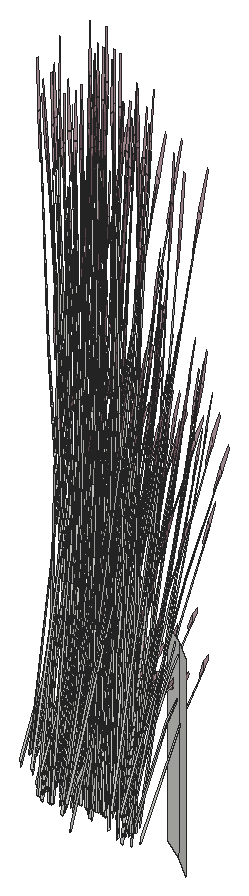
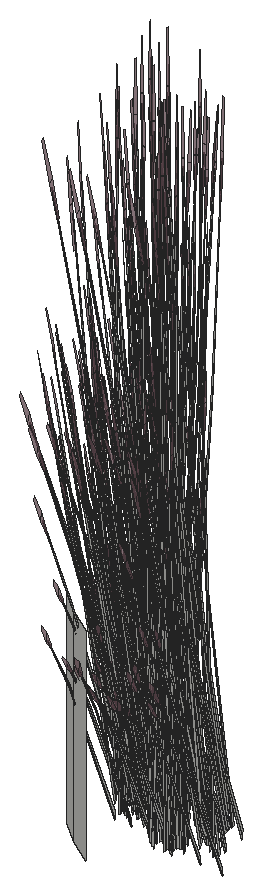
# SketchUp Ruby script. Lengths in inches.
U = 1.inch
M = Sketchup.active_model
def pt(a) = Geom::Point3d.new(a.map { |v| v * U })
def face(e, loops, mat)
  f = e.add_face(loops[0].map { |a| pt(a) })
  loops[1..].each { |l| e.add_face(l.map { |a| pt(a) }).erase! }
  f.material = f.back_material = mat if mat
  f
end
# faces: each face lists its corners as indices into pts; further lists are holes
def faces(e, pts, list, mat = nil) = list.each { |f| face(e, (f[0].is_a?(Array) ? f : [f]).map { |l| l.map { |i| pts[i] } }, mat) }
# xy, xz, yz: faces in a plane at the given z, y or x. An outline is a flat list of corners, or four numbers for a rectangle; further outlines are holes
def ring(l) = l.size == 4 ? [[l[0], l[1]], [l[2], l[1]], [l[2], l[3]], [l[0], l[3]]] : l.each_slice(2).to_a
def flat(e, list, mat, &to3) = list.each { |f| face(e, (f[0].is_a?(Array) ? f : [f]).map { |l| ring(l).map { |u, v| to3.(u, v) } }, mat) }
def xy(e, z, list, mat = nil) = flat(e, list, mat) { |x, y| [x, y, z] }
def xz(e, y, list, mat = nil) = flat(e, list, mat) { |x, z| [x, y, z] }
def yz(e, x, list, mat = nil) = flat(e, list, mat) { |y, z| [x, y, z] }
def lines(e, pts, list) = list.each { |a, b| e.add_line(pt(pts[a]), pt(pts[b])) }
# prism: a flat outline (further loops are holes) pulled along v
def prism(e, loops, v, mat = nil)
  f = face(e, loops, mat); d = Geom::Vector3d.new(v.map { |x| x * U })
  f.pushpull(f.normal.samedirection?(d) ? d.length : -d.length)
end
def box(e, o, s, mat = nil) = prism(e, [[o, [o[0] + s[0], o[1], o[2]], [o[0] + s[0], o[1] + s[1], o[2]], [o[0], o[1] + s[1], o[2]]]], [0, 0, s[2]], mat)
def at(x, y, z, deg = 0) = Geom::Transformation.translation(pt([x, y, z])) * Geom::Transformation.rotation(ORIGIN, Z_AXIS, deg.degrees)
def axes(o, x, y, z) = Geom::Transformation.new([*x, 0, *y, 0, *z, 0, *pt(o).to_a, 1])
def part(name) = M.definitions.add(name)
# library, detail: a bought-in or finely detailed component or shape, given as its bounding box
def library(name, o, s) = part(name).tap { |d| box(d.entities, o, s) }
def detail(e, o, s) = box(e.add_group.entities, o, s)
def put(e, d, t, mat = nil) = e.add_instance(d, t).tap { |i| i.material = mat if mat }
def group(e, t, mat = nil) = e.add_group.tap { |g| g.transformation = t; g.material = mat if mat }.entities
root = M.entities
M.materials.add("LightPink_Translucent").color = [144, 107, 117]
M.materials["LightPink_Translucent"].alpha = 0.75
c1 = part("blade")
p = [[2.15,0.21,22],[0,0.17,0],[0.09,0.45,0],[2.18,0.31,22],[2.29,0.31,22],[0.38,0.45,0],
  [2.48,0.24,33],[2.49,0.24,33],[2.48,0.22,33]]
faces(c1.entities,p,[[0,1,2,3],[4,5,2,3],[6,3,4,7],[8,0,3,6]])
c2 = part("seeds")
p = [[0.3,-0.1,1.38],[-0.01,-0.03,1.59],[-0.01,-0.03,0.03],[0.14,-0.07,-0.07],[0.29,-0.03,3],[0.15,0.01,3.11]]
faces(c2.entities,p,[[0,1,2,3],[1,0,4,5]],"LightPink_Translucent")
c3 = part("blade with seeds")
put(c3.entities,c1,at(0,0,0))
put(c3.entities,c2,axes([2.4,0.25,30.99],[1.5799,-0.05474,1.17369],[-0.12525,1.92788,0.29478],[-0.07173,-0.02425,1.56792]))
p = [[367.36,357.2,618],[369.42,355.39,618],[369.42,355.39,636],[367.36,357.2,636],[365.07,358.73,618],[365.07,358.73,636]]
faces(root,p,[[0,1,2,3],[4,0,3,5]])
put(root,c3,axes([354.65,355.82,623.05],[-0.20082,-0.29199,0.35414],[0.2293,-0.2764,-0.4572],[0.1165,0.04206,0.87481]))
put(root,c3,axes([355.86,357.4,623.65],[0.2439,-0.26754,-0.06488],[0.22348,0.29302,-0.29416],[0.01573,0.08303,0.97024]))
put(root,c3,axes([358.69,356.23,620.06],[-0.23773,0.35053,-0.62353],[-0.29532,-0.31785,-0.16365],[-0.09526,0.08744,1.37633]))
put(root,c3,axes([354.83,356.09,622.73],[-0.01777,0.35463,0.0643],[-0.26836,-0.00972,0.50621],[0.1028,0.03711,0.77189]))
put(root,c3,axes([358.5,356.01,622.73],[-0.08753,-0.42921,0.48003],[0.34336,-0.07449,0.3958],[-0.1012,0.10094,0.9933]))
put(root,c3,axes([356.14,355.7,620.2],[0.35581,0.20937,0],[-0.17124,0.43505,0],[0,0,1.74954]))
put(root,c3,axes([354.76,356.64,619.49],[0.02571,-0.06733,1.76342],[0.32373,-0.19829,-0.26939],[0.09815,0.10263,0.30037]))
put(root,c3,axes([354.86,355.98,622.73],[-0.26024,0.30729,0.48003],[-0.22444,-0.32634,0.3958],[0.1221,0.05668,0.9933]))
put(root,c3,axes([358.4375,355.93,622.73],[-0.2423,-0.19613,0.0643],[0.14107,-0.2793,0.50621],[-0.07768,0.0903,0.77189]))
put(root,c3,axes([358.85,356.03,620.46],[-0.34464,-0.37536,-0.25192],[0.29,-0.42149,0.5513],[-0.0928,0.04391,1.68216]))
put(root,c3,axes([357.19,354.89,620.03],[-0.24637,0.29097,-0.30978],[-0.24637,-0.29097,0.30978],[0,0.09372,1.38974]))
put(root,c3,axes([356.49,354.84,620.09],[0.12941,0.42699,-0.69212],[-0.37279,0.15378,-0.18165],[0.0143,0.14459,1.52773]))
put(root,c3,axes([358.68,355.95,620.21],[-0.38326,0.02879,-0.44739],[-0.03466,-0.47788,0.21531],[-0.06861,0.04843,1.43643]))
put(root,c3,axes([358.72,356.14,622.68],[0.09067,0.42583,-0.51099],[-0.34336,0.07449,-0.3958],[-0.0984,0.11438,0.97773]))
put(root,c3,axes([357.95,356.75,620.48],[0.33032,0.23318,0.49651],[-0.19744,0.41812,0],[-0.07523,-0.05311,1.57504]))
put(root,c3,axes([356.33,354.36,620.67],[0.39748,0.22252,-0.29095],[-0.19139,0.46966,-0.50002],[0.01249,0.11531,1.59708]))
put(root,c3,axes([354.22,355.23,621.875],[-0.1311,-0.08035,1.71376],[0.27131,-0.33708,0.13857],[0.16909,0.15206,0.73262]))
put(root,c3,axes([359.08,357.1875,620.02],[-0.33032,0.23318,-0.49651],[-0.19744,-0.41812,0],[-0.07523,0.05311,1.57504]))
put(root,c3,axes([359.1,357.0625,620.19],[-0.21791,-0.46895,-0.05142],[0.36918,-0.26061,0.51607],[-0.09097,0.04465,1.6363]))
put(root,c3,axes([357.36,354.9,620.02],[0,0.46636,-0.49651],[-0.39487,0,0],[0,0.10622,1.57504]))
put(root,c3,axes([356.31,356.32,622.73],[-0.35104,0.10702,0.48003],[-0.06092,-0.41983,0.3958],[0.08256,0.12373,0.9933]))
put(root,c3,axes([354.9375,355.98,622.53],[0.20082,0.29199,-0.35414],[-0.2293,0.2764,0.4572],[0.1165,0.04206,0.87481]))
put(root,c3,axes([356.24,356.4,622.73],[-0.16041,0.29625,0.0643],[-0.22843,-0.17248,0.50621],[0.07385,0.09498,0.77189]))
put(root,c3,axes([358.56,355.84,623.03],[0.32648,0.25715,-0.1216],[-0.18809,0.3724,-0.67495],[-0.09224,0.12945,1.02557]))
put(root,c3,axes([359,357,620.03],[-0.32928,-0.11539,-0.30978],[0.08291,-0.40636,0.30978],[-0.06638,0.04686,1.38974]))
put(root,c3,axes([357.59,356.62,623.05],[0.23881,-0.24554,0.35414],[0.22606,0.28036,-0.4572],[-0.0344,0.14245,0.87481]))
put(root,c3,axes([359.29,357.01,620.375],[-0.22066,0.46731,0],[-0.36918,-0.26061,-0.51607],[-0.08408,-0.05936,1.63711]))
put(root,c3,axes([358.02,356.95,623.65],[0.31145,0.12449,-0.06488],[-0.0958,0.38314,-0.29416],[-0.05094,0.05817,0.97024]))
put(root,c3,axes([358.95,355.82,620.67],[0.04113,0.53214,-0.29095],[-0.42835,0.03218,-0.50002],[-0.07543,0.07088,1.59708]))
put(root,c3,axes([358.71,355.87,623.05],[0.30722,-0.06665,0.35414],[0.08112,0.381,-0.4572],[-0.08804,0.10234,0.87481]))
put(root,c3,axes([355.02,355.73,622.72],[0.07571,-0.00789,1.74944],[0.20767,-0.36231,-0.27667],[0.13467,0.04783,0.14031]))
put(root,c3,axes([356.1875,356.06,623.05],[-0.05451,-0.37564,0.35414],[0.31161,-0.09919,-0.4572],[0.0837,0.10765,0.87481]))
put(root,c3,axes([356.4,353.9,622.47],[-0.30498,-0.24231,1.38283],[0.32203,-0.37727,0.59665],[0.0984,0.22736,1.33663]))
put(root,c3,axes([355.88,356.58,622.71],[0.00104,-0.05646,1.77383],[0.30246,-0.2491,-0.16761],[0.10506,0.08891,0.31391]))
put(root,c3,axes([356.86,355.87,620.77],[-0.19872,-0.13409,1.1486],[0.2566,-0.13625,0.84392],[0.06921,0.11541,0.25299]))
put(root,c3,axes([356.15,355.73,620.59],[0.00623,-0.15459,1.43002],[0.29764,-0.17268,-0.30754],[0.09188,0.18503,0.61141]))
put(root,c3,axes([354.73,355.78,622.98],[0.35281,0.01123,-0.71045],[-0.0237,0.47284,0.08574],[0.14947,0.0499,1.00501]))
put(root,c3,axes([358.56,356.59,620.2],[-0.35581,-0.20937,0],[0.17124,-0.43505,0],[0,0,1.62707]))
put(root,c3,axes([357.46,354.55,620.375],[0.44133,0,0],[0,0.52122,-0.51607],[0,0.11871,1.63711]))
put(root,c3,axes([360.23,356.24,620.06],[-0.23773,0.35053,-0.62353],[-0.29532,-0.31785,-0.16365],[-0.09526,0.08744,1.37633]))
put(root,c3,axes([359.38,357.11,620.375],[0.22066,0.46731,0],[-0.36918,0.26061,-0.51607],[-0.08408,0.05936,1.63711]))
put(root,c3,axes([359.41,353.62,620.59],[0.11138,-0.07357,1.43002],[0.27499,0.22183,-0.30754],[-0.08185,0.19194,0.61141]))
put(root,c3,axes([356.89,356.48,620.67],[-0.22633,-0.01463,1.0506],[0.14947,-0.31064,0.58006],[0.08941,0.11036,0.8241]))
put(root,c3,axes([359.03,355.93,620.62],[0.26075,0.2802,0.1448],[-0.2175,0.31612,-0.41347],[-0.06054,0.04274,1.26744]))
put(root,c3,axes([360.39,356.04,620.46],[-0.34464,-0.37536,-0.25192],[0.29,-0.42149,0.5513],[-0.0928,0.04391,1.68216]))
put(root,c3,axes([359.02,355.72,620.72],[0.38326,-0.02879,0.44739],[0.03466,0.47788,-0.21531],[-0.06861,0.04843,1.43643]))
put(root,c3,axes([359.11,356.82,620.33],[0.44186,0.15158,0.30756],[-0.11054,0.54181,-0.36492],[-0.07313,0.06781,1.64885]))
put(root,c3,axes([360.22,355.97,620.21],[-0.38326,0.02879,-0.44739],[-0.03466,-0.47788,0.21531],[-0.06861,0.04843,1.43643]))
put(root,c3,axes([356.16,356.25,623.03],[0.21031,-0.39918,-0.1216],[0.30457,0.22997,-0.67495],[0.10587,0.11278,1.02557]))
put(root,c3,axes([359.3,356.79,620.48],[0.33032,-0.23318,0.49651],[0.19744,0.41812,0],[-0.07523,0.05311,1.57504]))
put(root,c3,axes([355.51,355.55,620.59],[-0.085,-0.1147,1.43002],[0.1106,-0.37943,-0.30754],[0.17198,0.0514,0.61141]))
put(root,c3,axes([359.48,356.76,620.48],[0.33032,0.23318,0.49651],[-0.19744,0.41812,0],[-0.07523,-0.05311,1.57504]))
put(root,c3,axes([356.41,356.05,622.68],[0.34827,-0.11086,-0.51099],[0.06092,0.41983,-0.3958],[0.09354,0.12031,0.97773]))
put(root,c3,axes([358.68,353.78,622.71],[0.04004,-0.02816,1.77383],[0.33095,0.18728,-0.16761],[-0.00778,0.15594,0.31391]))
put(root,c3,axes([360.62,357.2,620.02],[-0.33032,0.23318,-0.49651],[-0.19744,-0.41812,0],[-0.07523,0.05311,1.57504]))
put(root,c3,axes([360.64,357.07,620.19],[-0.21791,-0.46895,-0.05142],[0.36918,-0.26061,0.51607],[-0.09097,0.04465,1.6363]))
put(root,c3,axes([356.99,355.82,622.73],[-0.01777,0.35463,0.0643],[-0.26836,-0.00972,0.50621],[0.1028,0.03711,0.77189]))
put(root,c3,axes([359.1,355.62,620.21],[-0.17124,0.42022,-0.44739],[-0.35581,-0.20224,0.21531],[0,0.09687,1.43643]))
put(root,c3,axes([356.91,356.37,619.49],[0.02571,-0.06733,1.76342],[0.32373,-0.19829,-0.26939],[0.09815,0.10263,0.30037]))
put(root,c3,axes([357.02,355.7,622.73],[-0.26024,0.30729,0.48003],[-0.22444,-0.32634,0.3958],[0.1221,0.05668,0.9933]))
put(root,c3,axes([359.6875,352.65,623.34],[-0.00918,0.43138,-0.7886],[-0.38672,-0.02897,0.09517],[-0.04081,0.18275,1.11556]))
put(root,c3,axes([360.54,357.01,620.03],[-0.32928,-0.11539,-0.30978],[0.08291,-0.40636,0.30978],[-0.06638,0.04686,1.38974]))
put(root,c3,axes([359.78,355.36,620.47],[-0.2773,-0.3397,0.17642],[0.27945,-0.32949,0.35086],[-0.03063,0.06937,1.60407]))
put(root,c3,axes([359.13,356.63,623.05],[0.23881,-0.24554,0.35414],[0.22606,0.28036,-0.4572],[-0.0344,0.14245,0.87481]))
put(root,c3,axes([359.05,355.38,620.29],[0,0.53934,-0.05637],[-0.44133,0,0],[0,0.01695,1.79368]))
put(root,c3,axes([358.83,356.42,620.29],[0.15345,0.53576,-0.06012],[-0.43845,0.18773,0],[0.00536,0.01871,1.72173]))
put(root,c3,axes([360.48,355.84,620.67],[0.04113,0.53214,-0.29095],[-0.42835,0.03218,-0.50002],[-0.07543,0.07088,1.59708]))
put(root,c3,axes([359.56,353.26,621.36],[0.00775,-0.24075,1.54345],[0.34877,0.12716,0.21329],[-0.03022,0.25658,0.72882]))
put(root,c3,axes([360.1,355.72,620.2],[-0.44111,-0.00373,-0.04976],[0,-0.52122,0.49943],[-0.01386,0.11865,1.58352]))
put(root,c3,axes([356.37,354.96,621.875],[-0.1311,-0.08035,1.71376],[0.27131,-0.33708,0.13857],[0.16909,0.15206,0.73262]))
put(root,c3,axes([359.76,352.79,623],[0.25266,0.31335,-0.5672],[-0.2669,0.27442,-0.43934],[-0.03844,0.15921,1.08528]))
put(root,c3,axes([359.11,355.49,620.21],[0.24637,0.30123,0],[-0.24637,0.30123,0],[0,0,1.69266]))
put(root,c3,axes([359.11,355.14,620.72],[0.17124,-0.42022,0.44739],[0.35581,0.20224,-0.21531],[0,0.09687,1.43643]))
put(root,c3,axes([358.96,356.6,620.2],[0.35581,0.20937,0],[-0.17124,0.43505,0],[0,0,1.74954]))
put(root,c3,axes([357.09,355.7,622.53],[0.20082,0.29199,-0.35414],[-0.2293,0.2764,0.4572],[0.1165,0.04206,0.87481]))
put(root,c3,axes([359.49,353.26,620.82],[0.32063,-0.08258,0.06507],[0.07371,0.33271,-0.86304],[-0.02033,0.16842,0.7736]))
put(root,c3,axes([360.01,355.8,620.03],[-0.24637,0.29097,-0.30978],[-0.24637,-0.29097,0.30978],[0,0.09372,1.38974]))
put(root,c3,axes([360.09,356.6,620.2],[-0.35581,-0.20937,0],[0.17124,-0.43505,0],[0,0,1.62707]))
put(root,c3,axes([360.05,352.34,621.875],[-0.00864,-0.17899,1.71376],[0.37441,0.11874,0.13857],[-0.02316,0.25508,0.73262]))
put(root,c3,axes([359.26,355.23,620.62],[0.32884,-0.136,0.1448],[0.11516,0.38837,-0.41347],[0,0.08547,1.26744]))
put(root,c3,axes([357.18,355.45,622.72],[0.07571,-0.00789,1.74944],[0.20767,-0.36231,-0.27667],[0.13467,0.04783,0.14031]))
put(root,c3,axes([360.5625,355.9375,620.62],[0.26075,0.2802,0.1448],[-0.2175,0.31612,-0.41347],[-0.06054,0.04274,1.26744]))
put(root,c3,axes([360.56,355.73,620.72],[0.38326,-0.02879,0.44739],[0.03466,0.47788,-0.21531],[-0.06861,0.04843,1.43643]))
put(root,c3,axes([359.15,355.27,620.67],[0.39748,0.22252,-0.29095],[-0.19139,0.46966,-0.50002],[0.01249,0.11531,1.59708]))
put(root,c3,axes([360.65,356.83,620.33],[0.44186,0.15158,0.30756],[-0.11054,0.54181,-0.36492],[-0.07313,0.06781,1.64885]))
put(root,c3,axes([360.84,356.8,620.48],[0.33032,-0.23318,0.49651],[0.19744,0.41812,0],[-0.07523,0.05311,1.57504]))
put(root,c3,axes([360.01,355.37,620.48],[0,-0.46636,0.49651],[0.39487,0,0],[0,0.10622,1.57504]))
put(root,c3,axes([356.88,355.51,622.98],[0.35281,0.01123,-0.71045],[-0.0237,0.47284,0.08574],[0.14947,0.0499,1.00501]))
put(root,c3,axes([360.18,355.81,620.02],[0,0.46636,-0.49651],[-0.39487,0,0],[0,0.10622,1.57504]))
put(root,c3,axes([360.64,355.63,620.21],[-0.17124,0.42022,-0.44739],[-0.35581,-0.20224,0.21531],[0,0.09687,1.43643]))
put(root,c3,axes([361.32,355.37,620.47],[-0.2773,-0.3397,0.17642],[0.27945,-0.32949,0.35086],[-0.03063,0.06937,1.60407]))
put(root,c3,axes([360.58,355.39,620.29],[0,0.53934,-0.05637],[-0.44133,0,0],[0,0.01695,1.79368]))
put(root,c3,axes([359.01,356.96,623.05],[-0.05451,-0.37564,0.35414],[0.31161,-0.09919,-0.4572],[0.0837,0.10765,0.87481]))
put(root,c3,axes([363.13,353.51,621.875],[0.08815,-0.14329,1.71376],[0.22258,0.38678,0.13857],[-0.15267,0.17614,0.73262]))
put(root,c3,axes([359.08,355,620.21],[0.21202,0.39143,-0.44739],[-0.32115,0.27564,0.21531],[0.06861,0.04843,1.43643]))
put(root,c3,axes([360.37,356.43,620.29],[0.15345,0.53576,-0.06012],[-0.43845,0.18773,0],[0.00536,0.01871,1.72173]))
put(root,c3,axes([360.28,353.2,619.49],[0.05712,-0.02538,1.76342],[0.34359,0.13968,-0.26939],[0.01005,0.15742,0.30037]))
put(root,c3,axes([362.43,355.01,619.49],[0.04734,0.04659,1.76342],[0.08027,0.4317,-0.26939],[-0.10492,0.09206,0.30037]))
put(root,c3,axes([359.22,354.8,622.47],[-0.30498,-0.24231,1.38283],[0.32203,-0.37727,0.59665],[0.0984,0.22736,1.33663]))
put(root,c3,axes([360.36,353.34,622.53],[-0.1064,0.35863,-0.35414],[-0.31043,-0.1046,0.4572],[0.02846,0.14439,0.87481]))
put(root,c3,axes([359.68,356.77,620.77],[-0.19872,-0.13409,1.1486],[0.2566,-0.13625,0.84392],[0.06921,0.11541,0.25299]))
put(root,c3,axes([361.64,355.73,620.2],[-0.44111,-0.00373,-0.04976],[0,-0.52122,0.49943],[-0.01386,0.11865,1.58352]))
put(root,c3,axes([360.28,355.45,620.375],[0.44133,0,0],[0,0.52122,-0.51607],[0,0.11871,1.63711]))
put(root,c3,axes([360.14,353.98,622.72],[0.04474,0.0751,1.74944],[0.36104,0.0295,-0.27667],[0.03631,0.16562,0.14031]))
put(root,c3,axes([360.65,355.5,620.21],[0.24637,0.30123,0],[-0.24637,0.30123,0],[0,0,1.69266]))
put(root,c3,axes([363.07,353.86,621.875],[0.06572,-0.16029,1.71376],[0.27569,0.33172,0.13857],[-0.12437,0.20675,0.73262]))
put(root,c3,axes([360.65,355.15,620.72],[0.17124,-0.42022,0.44739],[0.35581,0.20224,-0.21531],[0,0.09687,1.43643]))
put(root,c3,axes([360.5,356.61,620.2],[0.35581,0.20937,0],[-0.17124,0.43505,0],[0,0,1.74954]))
put(root,c3,axes([362.85,353.92,622.68],[0.09067,0.42583,-0.51099],[-0.34336,0.07449,-0.3958],[-0.0984,0.11438,0.97773]))
put(root,c3,axes([361.55,355.81,620.03],[-0.24637,0.29097,-0.30978],[-0.24637,-0.29097,0.30978],[0,0.09372,1.38974]))
put(root,c3,axes([362.32,354.69,622.72],[-0.00877,0.09229,1.74944],[0.24897,0.32105,-0.27667],[-0.06518,0.15182,0.14031]))
put(root,c3,axes([358.98,357.16,623.03],[0.21031,-0.39918,-0.1216],[0.30457,0.22997,-0.67495],[0.10587,0.11278,1.02557]))
put(root,c3,axes([360.39,353.02,622.98],[0.16845,0.3792,-0.71045],[-0.34676,0.21133,0.08574],[0.03939,0.18322,1.00501]))
put(root,c3,axes([360.8,355.25,620.62],[0.32884,-0.136,0.1448],[0.11516,0.38837,-0.41347],[0,0.08547,1.26744]))
put(root,c3,axes([360.68,355.28,620.67],[0.39748,0.22252,-0.29095],[-0.19139,0.46966,-0.50002],[0.01249,0.11531,1.59708]))
put(root,c3,axes([362.69,353.62,623.03],[0.32648,0.25715,-0.1216],[-0.18809,0.3724,-0.67495],[-0.09224,0.12945,1.02557]))
put(root,c3,axes([359.63,356.45,623.05],[-0.20082,-0.29199,0.35414],[0.2293,-0.2764,-0.4572],[0.1165,0.04206,0.87481]))
put(root,c3,axes([360.51,353.1,622.68],[0.34695,0.11691,-0.51099],[-0.11892,0.40083,-0.3958],[0.03181,0.16138,0.97773]))
put(root,c3,axes([359.8125,356.72,622.73],[-0.01777,0.35463,0.0643],[-0.26836,-0.00972,0.50621],[0.1028,0.03711,0.77189]))
put(root,c3,axes([359.84,356.61,622.73],[-0.26024,0.30729,0.48003],[-0.22444,-0.32634,0.3958],[0.1221,0.05668,0.9933]))
put(root,c3,axes([361.55,355.38,620.48],[0,-0.46636,0.49651],[0.39487,0,0],[0,0.10622,1.57504]))
put(root,c3,axes([361.72,355.82,620.02],[0,0.46636,-0.49651],[-0.39487,0,0],[0,0.10622,1.57504]))
put(root,c3,axes([362.15,354.74,623.65],[0.31145,0.12449,-0.06488],[-0.0958,0.38314,-0.29416],[-0.05094,0.05817,0.97024]))
put(root,c3,axes([360.51,356.65,621.93],[-0.06755,-0.39203,-0.03492],[0.31928,-0.09013,-0.15832],[0.06667,0.02485,0.52218]))
put(root,c3,axes([363.03,355.47,620.59],[0.11138,-0.07357,1.43002],[0.27499,0.22183,-0.30754],[-0.08185,0.19194,0.61141]))
put(root,c3,axes([359.27,354.85,620.06],[0.36714,0.07646,-0.62353],[-0.07747,0.47163,-0.16365],[0.10956,0.05715,1.37633]))
put(root,c3,axes([363.14,354.67,622.73],[-0.25132,-0.3182,0.48003],[0.2669,-0.27442,0.3958],[-0.04636,0.14929,0.9933]))
put(root,c3,axes([360.54,356.97,623.05],[-0.05451,-0.37564,0.35414],[0.31161,-0.09919,-0.4572],[0.0837,0.10765,0.87481]))
put(root,c3,axes([363.05,354.64,622.73],[-0.29004,-0.02173,0.0643],[0.00795,-0.32812,0.50621],[-0.03035,0.12569,0.77189]))
put(root,c3,axes([360.61,355.01,620.21],[0.21202,0.39143,-0.44739],[-0.32115,0.27564,0.21531],[0.06861,0.04843,1.43643]))
put(root,c3,axes([359.19,355.86,621.875],[-0.1311,-0.08035,1.71376],[0.27131,-0.33708,0.13857],[0.16909,0.15206,0.73262]))
put(root,c3,axes([363.14,354.76,622.53],[-0.23881,0.24554,-0.35414],[-0.22606,-0.28036,0.4572],[-0.0344,0.14245,0.87481]))
put(root,c3,axes([360.75,354.8125,622.47],[-0.30498,-0.24231,1.38283],[0.32203,-0.37727,0.59665],[0.0984,0.22736,1.33663]))
put(root,c3,axes([360.71,352.27,621.875],[-0.08068,-0.14973,1.71376],[0.3728,-0.12606,0.13857],[0.08426,0.23506,0.73262]))
put(root,c3,axes([361.21,356.79,620.77],[-0.19872,-0.13409,1.1486],[0.2566,-0.13625,0.84392],[0.06921,0.11541,0.25299]))
put(root,c3,axes([364.36,354.03,620.06],[-0.23773,0.35053,-0.62353],[-0.29532,-0.31785,-0.16365],[-0.09526,0.08744,1.37633]))
put(root,c3,axes([359.91,356.61,622.53],[0.20082,0.29199,-0.35414],[-0.2293,0.2764,0.4572],[0.1165,0.04206,0.87481]))
put(root,c3,axes([362.29,355.64,622.71],[0.04004,-0.02816,1.77383],[0.33095,0.18728,-0.16761],[-0.00778,0.15594,0.31391]))
put(root,c3,axes([359.68,356.64,623.03],[0.0189,-0.47427,-0.1216],[0.35781,0.01296,-0.67495],[0.13781,0.03295,1.02557]))
put(root,c3,axes([361.8125,355.46,620.375],[0.44133,0,0],[0,0.52122,-0.51607],[0,0.11871,1.63711]))
put(root,c3,axes([363.3,354.5,623.34],[-0.00918,0.43138,-0.7886],[-0.38672,-0.02897,0.09517],[-0.04081,0.18275,1.11556]))
put(root,c3,axes([363.29,355.72,620.77],[-0.00913,-0.2773,1.1486],[0.22824,0.19778,0.84392],[-0.04489,0.13217,0.25299]))
put(root,c3,axes([360,356.35,622.72],[0.07571,-0.00789,1.74944],[0.20767,-0.36231,-0.27667],[0.13467,0.04783,0.14031]))
put(root,c3,axes([360.89,355.67,620.77],[-0.21807,0.07699,1.1486],[0.10265,-0.31819,0.84392],[0.11568,0.02177,0.25299]))
put(root,c3,axes([360.52,357.17,623.03],[0.21031,-0.39918,-0.1216],[0.30457,0.22997,-0.67495],[0.10587,0.11278,1.02557]))
put(root,c3,axes([364.76,354.98,620.02],[-0.33032,0.23318,-0.49651],[-0.19744,-0.41812,0],[-0.07523,0.05311,1.57504]))
put(root,c3,axes([359.7,356.41,622.98],[0.35281,0.01123,-0.71045],[-0.0237,0.47284,0.08574],[0.14947,0.0499,1.00501]))
put(root,c3,axes([363.38,354.65,623],[0.25266,0.31335,-0.5672],[-0.2669,0.27442,-0.43934],[-0.03844,0.15921,1.08528]))
put(root,c3,axes([361.17,356.47,623.05],[-0.20082,-0.29199,0.35414],[0.2293,-0.2764,-0.4572],[0.1165,0.04206,0.87481]))
put(root,c3,axes([360.79,357.02,622.71],[-0.03191,-0.04083,1.77383],[0.06981,-0.43764,-0.16761],[0.12571,-0.02796,0.31391]))
put(root,c3,axes([363.27,354.41,623.05],[0.23881,-0.24554,0.35414],[0.22606,0.28036,-0.4572],[-0.0344,0.14245,0.87481]))
put(root,c3,axes([364.87,353.0625,620.84],[-0.00964,-0.43909,1.41272],[0.43635,0.11382,0.59816],[-0.1032,0.24027,1.3335]))
put(root,c3,axes([361.35,356.73,622.73],[-0.01777,0.35463,0.0643],[-0.26836,-0.00972,0.50621],[0.1028,0.03711,0.77189]))
put(root,c3,axes([361.37,356.62,622.73],[-0.26024,0.30729,0.48003],[-0.22444,-0.32634,0.3958],[0.1221,0.05668,0.9933]))
put(root,c3,axes([363.11,354.48,623.4],[0.3879,0.02311,-0.13498],[-0.0106,0.43749,-0.74919],[-0.02694,0.1685,1.13838]))
put(root,c3,axes([363.11,355.12,620.82],[0.32063,-0.08258,0.06507],[0.07371,0.33271,-0.86304],[-0.02033,0.16842,0.7736]))
put(root,c3,axes([362.05,356.66,621.93],[-0.06755,-0.39203,-0.03492],[0.31928,-0.09013,-0.15832],[0.06667,0.02485,0.52218]))
put(root,c3,axes([360.8,354.86,620.06],[0.36714,0.07646,-0.62353],[-0.07747,0.47163,-0.16365],[0.10956,0.05715,1.37633]))
put(root,c3,axes([363.67,354.2,621.875],[-0.00864,-0.17899,1.71376],[0.37441,0.11874,0.13857],[-0.02316,0.25508,0.73262]))
put(root,c3,axes([360.48,356.18,620.59],[-0.085,-0.1147,1.43002],[0.1106,-0.37943,-0.30754],[0.17198,0.0514,0.61141]))
put(root,c3,axes([360.73,355.87,621.875],[-0.1311,-0.08035,1.71376],[0.27131,-0.33708,0.13857],[0.16909,0.15206,0.73262]))
put(root,c3,axes([365.06,354.91,620.375],[0.22066,0.46731,0],[-0.36918,0.26061,-0.51607],[-0.08408,0.05936,1.63711]))
put(root,c3,axes([361.45,356.62,622.53],[0.20082,0.29199,-0.35414],[-0.2293,0.2764,0.4572],[0.1165,0.04206,0.87481]))
put(root,c3,axes([361.22,356.65,623.03],[0.0189,-0.47427,-0.1216],[0.35781,0.01296,-0.67495],[0.13781,0.03295,1.02557]))
put(root,c3,axes([363.93,355.11,623.0625],[-0.34777,-0.12192,0.53283],[0.11892,-0.40083,0.43934],[0.0209,0.15763,1.10256]))
put(root,c3,axes([363.84,355.14,622.73],[-0.26007,0.1585,0.0643],[-0.12729,-0.28902,0.50621],[0.02512,0.1274,0.77189]))
put(root,c3,axes([364.79,354.62,620.33],[0.44186,0.15158,0.30756],[-0.11054,0.54181,-0.36492],[-0.07313,0.06781,1.64885]))
put(root,c3,axes([361.53,356.37,622.72],[0.07571,-0.00789,1.74944],[0.20767,-0.36231,-0.27667],[0.13467,0.04783,0.14031]))
put(root,c3,axes([362.43,355.68,620.77],[-0.21807,0.07699,1.1486],[0.10265,-0.31819,0.84392],[0.11568,0.02177,0.25299]))
put(root,c3,axes([363.89,355.05,619.49],[0.05712,-0.02538,1.76342],[0.34359,0.13968,-0.26939],[0.01005,0.15742,0.30037]))
put(root,c3,axes([363.97,355.2,622.53],[-0.1064,0.35863,-0.35414],[-0.31043,-0.1046,0.4572],[0.02846,0.14439,0.87481]))
put(root,c3,axes([361.24,356.42,622.98],[0.35281,0.01123,-0.71045],[-0.0237,0.47284,0.08574],[0.14947,0.0499,1.00501]))
put(root,c3,axes([362.33,357.03,622.71],[-0.03191,-0.04083,1.77383],[0.06981,-0.43764,-0.16761],[0.12571,-0.02796,0.31391]))
put(root,c3,axes([363.9375,354.82,623.05],[0.1064,-0.35863,0.35414],[0.31043,0.1046,-0.4572],[0.02846,0.14439,0.87481]))
put(root,c3,axes([364,354.875,622.98],[0.16845,0.3792,-0.71045],[-0.34676,0.21133,0.08574],[0.03939,0.18322,1.00501]))
put(root,c3,axes([362.02,356.19,620.59],[-0.085,-0.1147,1.43002],[0.1106,-0.37943,-0.30754],[0.17198,0.0514,0.61141]))
put(root,c3,axes([364.35,356.1,623.65],[0.2439,-0.26754,-0.06488],[0.22348,0.29302,-0.29416],[0.01573,0.08303,0.97024]))
put(root,c3,axes([364.13,354.95,622.68],[0.34695,0.11691,-0.51099],[-0.11892,0.40083,-0.3958],[0.03181,0.16138,0.97773]))
put(root,c3,axes([363.83,354.97,623.03],[0.34538,-0.21713,-0.1216],[0.16972,0.38536,-0.67495],[0.04557,0.16239,1.02557]))
put(root,c3,axes([364.98,353.54,620.09],[0.12941,0.42699,-0.69212],[-0.37279,0.15378,-0.18165],[0.0143,0.14459,1.52773]))
put(root,c3,axes([365.85,353.6,620.02],[0,0.46636,-0.49651],[-0.39487,0,0],[0,0.10622,1.57504]))
put(root,c3,axes([364.8,355.02,622.73],[-0.35104,0.10702,0.48003],[-0.06092,-0.41983,0.3958],[0.08256,0.12373,0.9933]))
put(root,c3,axes([364.73,355.1,622.73],[-0.16041,0.29625,0.0643],[-0.22843,-0.17248,0.50621],[0.07385,0.09498,0.77189]))
put(root,c3,axes([364.33,354.12,621.875],[-0.08068,-0.14973,1.71376],[0.3728,-0.12606,0.13857],[0.08426,0.23506,0.73262]))
put(root,c3,axes([364.68,354.76,623.05],[-0.05451,-0.37564,0.35414],[0.31161,-0.09919,-0.4572],[0.0837,0.10765,0.87481]))
put(root,c3,axes([364.89,352.6,622.47],[-0.30498,-0.24231,1.38283],[0.32203,-0.37727,0.59665],[0.0984,0.22736,1.33663]))
put(root,c3,axes([364.38,355.28,622.71],[0.00104,-0.05646,1.77383],[0.30246,-0.2491,-0.16761],[0.10506,0.08891,0.31391]))
put(root,c3,axes([365.35,354.57,620.77],[-0.19872,-0.13409,1.1486],[0.2566,-0.13625,0.84392],[0.06921,0.11541,0.25299]))
put(root,c3,axes([364.64,354.43,620.59],[0.00623,-0.15459,1.43002],[0.29764,-0.17268,-0.30754],[0.09188,0.18503,0.61141]))
put(root,c3,axes([365.38,355.18,620.67],[-0.22633,-0.01463,1.0506],[0.14947,-0.31064,0.58006],[0.08941,0.11036,0.8241]))
put(root,c3,axes([364.65,354.95,623.03],[0.21031,-0.39918,-0.1216],[0.30457,0.22997,-0.67495],[0.10587,0.11278,1.02557]))
put(root,c3,axes([364.9,354.75,622.68],[0.34827,-0.11086,-0.51099],[0.06092,0.41983,-0.3958],[0.09354,0.12031,0.97773]))
put(root,c3,axes([365.41,355.07,619.49],[0.02571,-0.06733,1.76342],[0.32373,-0.19829,-0.26939],[0.09815,0.10263,0.30037]))
put(root,c3,axes([364.87,353.66,621.875],[-0.1311,-0.08035,1.71376],[0.27131,-0.33708,0.13857],[0.16909,0.15206,0.73262]))
